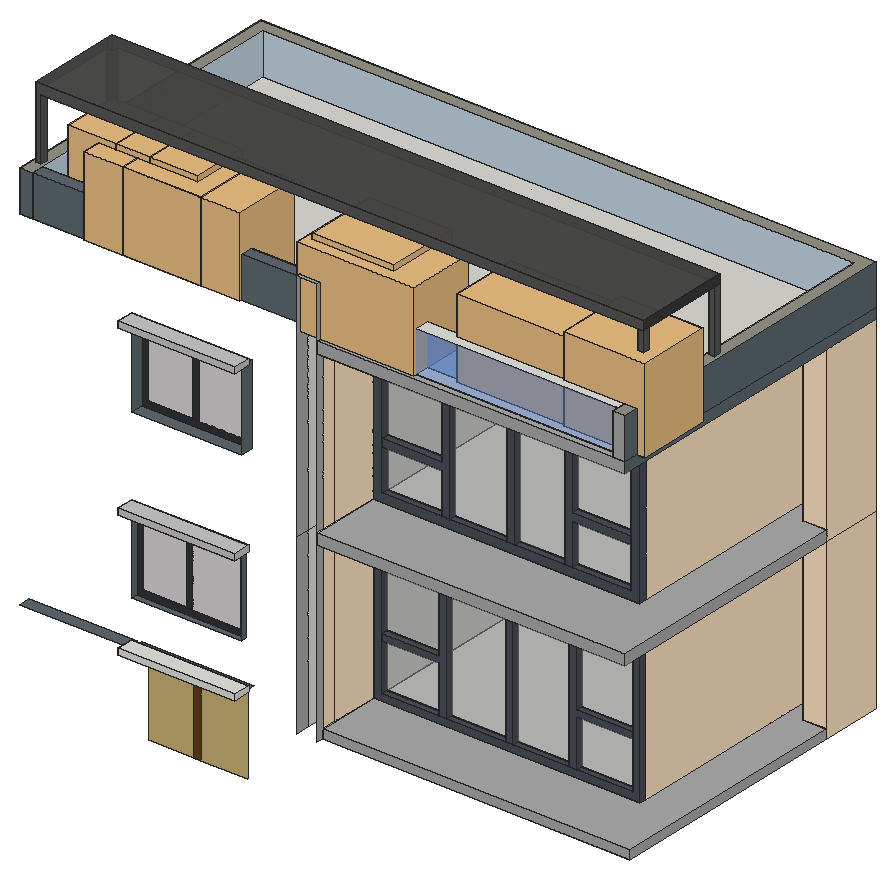
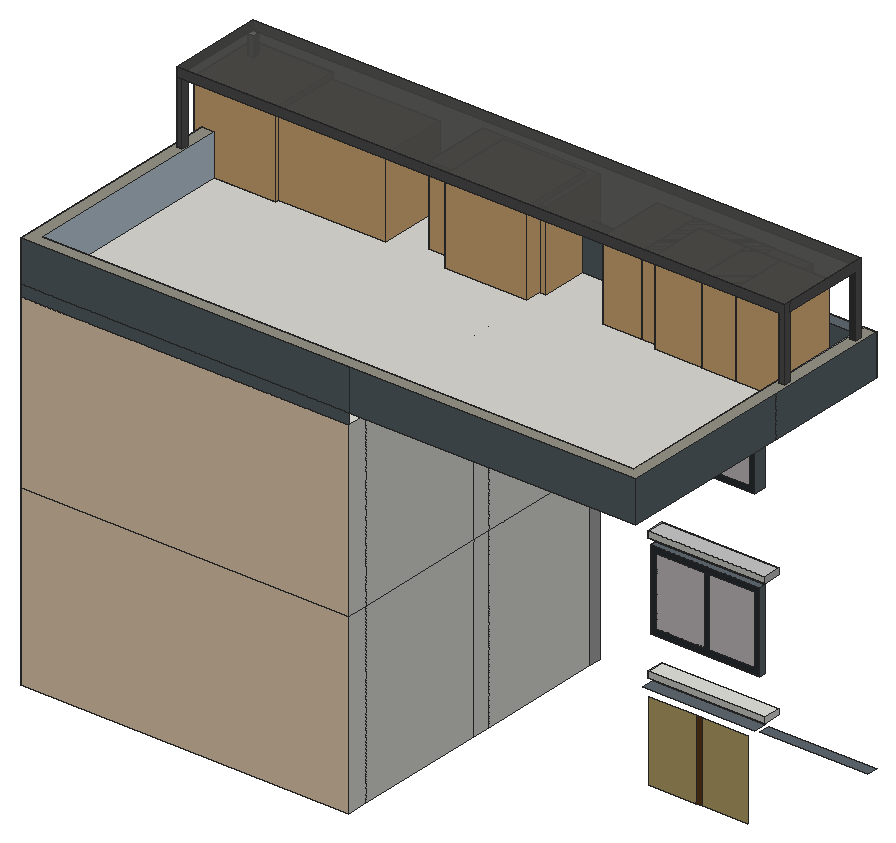
# SketchUp Ruby script. Lengths in inches.
U = 1.inch
M = Sketchup.active_model
def pt(a) = Geom::Point3d.new(a.map { |v| v * U })
def face(e, loops, mat)
  f = e.add_face(loops[0].map { |a| pt(a) })
  loops[1..].each { |l| e.add_face(l.map { |a| pt(a) }).erase! }
  f.material = f.back_material = mat if mat
  f
end
# faces: each face lists its corners as indices into pts; further lists are holes
def faces(e, pts, list, mat = nil) = list.each { |f| face(e, (f[0].is_a?(Array) ? f : [f]).map { |l| l.map { |i| pts[i] } }, mat) }
# xy, xz, yz: faces in a plane at the given z, y or x. An outline is a flat list of corners, or four numbers for a rectangle; further outlines are holes
def ring(l) = l.size == 4 ? [[l[0], l[1]], [l[2], l[1]], [l[2], l[3]], [l[0], l[3]]] : l.each_slice(2).to_a
def flat(e, list, mat, &to3) = list.each { |f| face(e, (f[0].is_a?(Array) ? f : [f]).map { |l| ring(l).map { |u, v| to3.(u, v) } }, mat) }
def xy(e, z, list, mat = nil) = flat(e, list, mat) { |x, y| [x, y, z] }
def xz(e, y, list, mat = nil) = flat(e, list, mat) { |x, z| [x, y, z] }
def yz(e, x, list, mat = nil) = flat(e, list, mat) { |y, z| [x, y, z] }
def lines(e, pts, list) = list.each { |a, b| e.add_line(pt(pts[a]), pt(pts[b])) }
# prism: a flat outline (further loops are holes) pulled along v
def prism(e, loops, v, mat = nil)
  f = face(e, loops, mat); d = Geom::Vector3d.new(v.map { |x| x * U })
  f.pushpull(f.normal.samedirection?(d) ? d.length : -d.length)
end
def box(e, o, s, mat = nil) = prism(e, [[o, [o[0] + s[0], o[1], o[2]], [o[0] + s[0], o[1] + s[1], o[2]], [o[0], o[1] + s[1], o[2]]]], [0, 0, s[2]], mat)
def at(x, y, z, deg = 0) = Geom::Transformation.translation(pt([x, y, z])) * Geom::Transformation.rotation(ORIGIN, Z_AXIS, deg.degrees)
def axes(o, x, y, z) = Geom::Transformation.new([*x, 0, *y, 0, *z, 0, *pt(o).to_a, 1])
def part(name) = M.definitions.add(name)
# library, detail: a bought-in or finely detailed component or shape, given as its bounding box
def library(name, o, s) = part(name).tap { |d| box(d.entities, o, s) }
def detail(e, o, s) = box(e.add_group.entities, o, s)
def put(e, d, t, mat = nil) = e.add_instance(d, t).tap { |i| i.material = mat if mat }
def group(e, t, mat = nil) = e.add_group.tap { |g| g.transformation = t; g.material = mat if mat }.entities
root = M.entities
M.materials.add("[0012_Bisque]").color = [255, 228, 196]
M.materials.add("[0035_Tan]").color = [210, 180, 140]
M.materials.add("[Blinds Cellular White]").color = [217, 211, 213]
M.materials.add("[Color M02]").color = [198, 198, 198]
M.materials.add("[Color M03]").color = [170, 170, 170]
M.materials.add("[Color M06]").color = [86, 86, 86]
M.materials.add("[Color M07]").color = [58, 58, 58]
M.materials.add("[Formica Graystone]1").color = [149, 146, 135]
M.materials.add("[Formica Laminate Dark]").color = [74, 78, 89]
M.materials.add("[Formica Speckled Grey]").color = [47, 53, 56]
M.materials.add("[Formica Speckled Grey]1").color = [94, 105, 111]
M.materials.add("[Terrazzo Light Blue]").color = [196, 214, 227]
M.materials.add("[Terrazzo Tile Light]").color = [219, 217, 210]
M.materials.add("[Translucent Glass Block Dark]1").color = [71, 71, 69]
M.materials["[Translucent Glass Block Dark]1"].alpha = 0.8
M.materials.add("[Translucent Glass Blue]").color = [100, 149, 237]
M.materials["[Translucent Glass Blue]"].alpha = 0.5
M.materials.add("[Translucent Glass Gray]1").color = [173, 173, 173]
M.materials["[Translucent Glass Gray]1"].alpha = 0.5
M.materials.add("[Window Covering 02]").color = [199, 178, 115]
M.materials.add("[Wood Floor Light]").color = [204, 176, 127]
M.materials.add("[Wood Floor Parquet]").color = [102, 62, 27]
M.materials.add("[Wood Floor]").color = [127, 86, 50]
c1 = library("chau cay",[-24.34,-109.24,0],[56.46,62.58,79.69])
c2 = library("Sem+nome",[-20.92,-6.25,0],[92.79,42.83,52.11])
box(root,[934.42,1163.08,1113.51],[394.37,58.44,20.12])
xy(root,972.31,[[2038.61,1644.77,2328.14,1674.71]],"[Wood Floor]")
xy(root,1077.79,[[1597.41,1197.49,1985.07,1247.68],[1597.41,1644.77,2438.87,2162.77]])
xy(root,1077.79,[[1985.07,1197.49,1985.07,1247.68,1597.41,1247.68,1597.41,1644.77,2438.87,1644.77,2438.87,2162.77,2570.48,2162.77,2570.48,2027.6,2634.5,2027.6,2634.5,1197.49]],"[0035_Tan]")
xy(root,1104.69,[[1597.41,1434.77,2496.41,2162.77],[2553.96,2027.6,2570.48,2162.77]])
xy(root,1106.33,[[1597.41,1413.09,2496.41,1434.77]])
xy(root,1106.33,[[1597.41,1197.49,2634.5,1197.49,2634.5,2027.6,2553.96,2027.6,2553.96,2162.77,2496.41,2162.77,2496.41,1413.09,1597.41,1413.09]],"[Color M03]")
xy(root,1108.67,[[560.3125,1221.52,922.73,1257.65],[937.5625,1221.52,1314.8125,1263.33]],"[Formica Speckled Grey]1")
xy(root,1129.41,[[1818.32,1413.09,1843.06,1434.77],[2042.55,1413.09,2067.28,1434.77],[2256.82,1413.09,2281.55,1434.77]])
xy(root,1129.41,[[1624.23,1413.09,1818.32,1434.77],[1843.06,1413.09,2042.55,1434.77],[2067.28,1413.09,2256.82,1434.77],[2281.55,1413.09,2469.59,1434.77]],"[Formica Laminate Dark]")
xy(root,1262.3,[[937.5625,1221.52,1307.26,1238.71]],"[Formica Speckled Grey]1")
xy(root,1288.71,[[1624.23,1413.09,1818.32,1434.77],[2281.55,1413.09,2469.59,1434.77]],"[Formica Laminate Dark]")
xy(root,1310.79,[[1624.23,1413.09,1818.32,1434.77],[2281.55,1413.09,2469.59,1434.77]],"[Formica Laminate Dark]")
xy(root,1522.7,[[1624.23,1413.09,1818.32,1434.77],[1843.06,1413.09,2042.55,1434.77],[2067.28,1413.09,2256.82,1434.77],[2281.55,1413.09,2469.59,1434.77]],"[Formica Laminate Dark]")
xy(root,1530.73,[[937.5625,1221.52,1307.26,1238.71]],"[Formica Speckled Grey]1")
xy(root,1536.95,[[934.42,1163.08,1328.79,1221.52]],"[Color M02]")
xy(root,1547.94,[[1624.23,1413.09,1818.32,1434.77],[1843.06,1413.09,2042.55,1434.77],[2067.28,1413.09,2256.82,1434.77],[2281.55,1413.09,2469.59,1434.77]],"[Formica Laminate Dark]")
xy(root,1557.07,[[934.42,1163.08,1328.79,1221.52]],"[Color M02]")
xy(root,1646.85,[[1818.32,1413.09,1843.06,1434.77],[2042.55,1413.09,2067.28,1434.77],[2256.82,1413.09,2281.55,1434.77]])
xy(root,1646.85,[[1624.23,1413.09,1818.32,1434.77],[1843.06,1413.09,2042.55,1434.77],[2067.28,1413.09,2256.82,1434.77],[2281.55,1413.09,2469.59,1434.77]],"[Formica Laminate Dark]")
xy(root,1671.57,[[1597.41,1413.09,2496.41,1434.77],[1597.41,1434.77,2496.41,2162.77]])
xy(root,1671.57,[[1597.41,1175.74,1597.41,1413.09,2496.41,1413.09,2496.41,2162.77,2553.96,2162.77,2553.96,2027.6,2634.5,2027.6,2634.5,1175.74]],"[0035_Tan]")
xy(root,1708.37,[[1597.41,1411.27,2496.41,1434.77],[1597.41,1434.77,2496.41,2162.77]])
xy(root,1708.37,[[1597.41,1175.74,2634.5,1175.74,2634.5,2027.6,2553.96,2027.6,2553.96,2162.77,2496.41,2162.77,2496.41,1411.27,1597.41,1411.27]],"[Color M03]")
xy(root,1736.45,[[1829.47,1411.27,1855.4,1434.77],[2047.9,1411.27,2073.84,1434.77],[2243.95,1411.27,2269.89,1434.77]])
xy(root,1736.45,[[1627.89,1411.27,1829.47,1434.77],[1855.4,1411.27,2047.9,1434.77],[2073.84,1411.27,2243.95,1434.77],[2269.89,1411.27,2465.9375,1434.77]],"[Formica Laminate Dark]")
xy(root,1822.8,[[937.5625,1221.52,1307.26,1262.83]],"[Formica Speckled Grey]1")
xy(root,1875.68,[[1627.89,1411.27,1829.47,1434.77],[2269.89,1411.27,2465.9375,1434.77]],"[Formica Laminate Dark]")
xy(root,1902.64,[[1627.89,1411.27,1829.47,1434.77],[2269.89,1411.27,2465.9375,1434.77]],"[Formica Laminate Dark]")
xy(root,2091.23,[[937.5625,1221.52,1307.26,1262.83]],"[Formica Speckled Grey]1")
xy(root,2100.86,[[1627.89,1411.27,1829.47,1434.77],[1855.4,1411.27,2047.9,1434.77],[2073.84,1411.27,2243.95,1434.77],[2269.89,1411.27,2465.9375,1434.77]],"[Formica Laminate Dark]")
xy(root,2101.01,[[934.42,1163.08,1328.79,1221.52]],"[Color M02]")
xy(root,2121.13,[[934.42,1163.08,1328.79,1221.52]],"[Color M02]")
xy(root,2123.1,[[1627.89,1411.27,1829.47,1434.77],[1855.4,1411.27,2047.9,1434.77],[2073.84,1411.27,2243.95,1434.77],[2269.89,1411.27,2465.9375,1434.77]],"[Formica Laminate Dark]")
xy(root,2222.77,[[1829.47,1411.27,1855.4,1434.77],[2047.9,1411.27,2073.84,1434.77],[2243.95,1411.27,2269.89,1434.77]])
xy(root,2222.77,[[1627.89,1411.27,1829.47,1434.77],[1855.4,1411.27,2047.9,1434.77],[2073.84,1411.27,2243.95,1434.77],[2269.89,1411.27,2465.9375,1434.77]],"[Formica Laminate Dark]")
xy(root,2250.85,[[1529,1256.68,1597.41,1434.77],[1597.41,1411.27,2496.41,1434.77],[1529,1434.77,1597.41,2234.7],[1597.41,1434.77,2496.41,2162.77],[2553.96,2027.6,2634.5,2234.7],
  [1597.41,2162.77,2438.87,2234.7],[2438.87,2162.77,2496.41,2234.7],[2496.41,2162.77,2553.96,2234.7]])
xy(root,2250.85,[[1597.41,1175.74,1597.41,1411.27,2496.41,1411.27,2496.41,2162.77,2553.96,2162.77,2553.96,2027.6,2634.5,2027.6,2634.5,1175.74]],"[0035_Tan]")
xy(root,2288.72,[[2592.99,1175.74,2592.99,2193.19,601.82,2193.19,601.82,1221.52,560.3125,1221.52,560.3125,2234.7,2634.5,2234.7,2634.5,1175.74],[1597.41,1197.49,2592.99,1243.8125],[601.82,1221.52,1529,1263.03],[1529,1247.68,1597.41,1256.68]])
xy(root,2288.72,[[1597.41,1175.74,2592.99,1197.49]],"[Color M03]")
xy(root,2288.72,[[1597.41,1243.8125,2592.99,1243.8125,2592.99,2193.19,601.82,2193.19,601.82,1263.03,1529,1263.03,1529,1256.68,1597.41,1256.68]],"[Terrazzo Tile Light]")
xy(root,2427.41,[[1597.41,1197.49,2592.99,1243.8125],[571.02,1271.52,590.77,1294.27],[2601.14,1271.52,2620.89,1294.27],[571.02,1571.45,590.77,1594.2],[2601.14,1571.45,2620.89,1594.2]])
xy(root,2427.41,[[[2592.99,1175.74,2634.5,1175.74,2634.5,2234.7,560.3125,2234.7,560.3125,1221.52,601.82,1221.52,601.82,2193.19,2592.99,2193.19],[2601.14,1271.52,2620.89,1294.27],[2601.14,1571.45,2620.89,1594.2],[571.02,1571.45,590.77,1594.2],[571.02,1271.52,590.77,1294.27]]],"[Formica Graystone]1")
xy(root,2427.41,[[601.82,1221.52,1529,1263.03]],"[Formica Speckled Grey]1")
xy(root,2461.1,[[1529,1175.74,1597.41,1247.68]],"[Color M03]")
xy(root,2636.87,[[2601.14,1271.52,2620.89,1294.27],[2601.14,1571.45,2620.89,1594.2]])
xy(root,2636.87,[[590.77,1271.52,590.77,1294.27,571.02,1294.27,571.02,1571.45,590.77,1571.45,590.77,1594.2,2601.14,1594.2,2601.14,1571.45,2620.89,1571.45,2620.89,1294.27,2601.14,1294.27,2601.14,1271.52]],"[Translucent Glass Block Dark]1")
xy(root,2667.72,[[571.02,1271.52,2620.89,1594.2]],"[Translucent Glass Block Dark]1")
xz(root,1163.08,[[934.42,1536.95,1328.79,1557.07],[934.42,2101.01,1328.79,2121.13]],"[Color M02]")
xz(root,1175.74,[[1597.41,1671.57,2634.5,1708.37],[1597.41,2250.85,2634.5,2288.72],[2592.99,2288.72,2634.5,2427.41]],"[Color M03]")
xz(root,1197.49,[[2586.03,2288.72,2592.99,2427.41]])
xz(root,1197.49,[[1597.41,1077.79,2634.5,1106.33]],"[Color M03]")
xz(root,1197.49,[[1597.41,2288.72,2586.03,2427.41]],"[Translucent Glass Blue]")
xz(root,1221.52,[[934.42,1536.95,1328.79,1557.07],[934.42,2101.01,1328.79,2121.13]])
xz(root,1221.52,[[560.3125,2288.72,601.82,2427.41],[601.82,2288.72,1529,2427.41]],"[Formica Speckled Grey]1")
xz(root,1238.71,[[958.89,1283.625,1106.3,1509.4],[1127,1283.625,1285.9375,1509.4]],"[Blinds Cellular White]")
xz(root,1238.71,[[[937.5625,1262.3,1307.26,1530.73],[958.89,1283.625,1285.9375,1509.4]],[1106.3,1283.625,1127,1509.4]],"[Formica Speckled Grey]")
xz(root,1243.8125,[[1597.41,2288.72,2592.99,2427.41]],"[Translucent Glass Blue]")
xz(root,1247.68,[[1529,2288.72,1597.41,2461.1]],"[Color M03]")
xz(root,1256.68,[[1529,2250.85,1597.41,2288.72]])
xz(root,1262.83,[[958.26,1843.5,1109,2070.53],[1133.75,1843.5,1286.57,2070.53]],"[Blinds Cellular White]")
xz(root,1262.83,[[[937.5625,1822.8,1307.26,2091.23],[958.26,1843.5,1286.57,2070.53]],[1109,1843.5,1133.75,2070.53]],"[Formica Speckled Grey]")
xz(root,1263.03,[[601.82,2288.72,1529,2427.41]],"[Formica Speckled Grey]1")
xz(root,1263.33,[[959.46,820.51,1112.13,1086.78],[1133.85,820.51,1292.91,1086.78]],"[Window Covering 02]")
xz(root,1263.33,[[1112.13,820.51,1133.85,1086.78]],"[Wood Floor Parquet]")
xz(root,1271.52,[[571.02,2427.41,590.77,2427.41,590.77,2636.87,2620.89,2636.87,2620.89,2667.72,571.02,2667.72],[2601.14,2427.41,2620.89,2636.87]],"[Color M06]")
xz(root,1294.27,[[2601.14,2427.41,2620.89,2636.87]])
xz(root,1294.27,[[571.02,2427.41,590.77,2636.87]],"[Color M07]")
xz(root,1411.27,[[[1597.41,1708.37,2496.41,2250.85],[1627.89,1736.45,2465.9375,2222.77]],[1829.47,1736.45,1855.4,1736.45,1855.4,2100.86,2047.9,2100.86,2047.9,1736.45,2073.84,1736.45,2073.84,2100.86,2243.95,2100.86,2243.95,1736.45,2269.89,1736.45,2269.89,1875.68,2465.9375,1875.68,2465.9375,1902.64,2269.89,1902.64,2269.89,2100.86,2465.9375,2100.86,2465.9375,2123.1,2269.89,2123.1,2269.89,2222.77,2243.95,2222.77,2243.95,2123.1,2073.84,2123.1,2073.84,2222.77,2047.9,2222.77,2047.9,2123.1,1855.4,2123.1,1855.4,2222.77,1829.47,2222.77,1829.47,2123.1,1627.89,2123.1,1627.89,2100.86,1829.47,2100.86,1829.47,1902.64,1627.89,1902.64,1627.89,1875.68,1829.47,1875.68]],"[Formica Laminate Dark]")
xz(root,1413.09,[[[1597.41,1106.33,2496.41,1671.57],[1624.23,1129.41,2469.59,1646.85]],[1818.32,1129.41,1843.06,1129.41,1843.06,1522.7,2042.55,1522.7,2042.55,1129.41,2067.28,1129.41,2067.28,1522.7,2256.82,1522.7,2256.82,1129.41,2281.55,1129.41,2281.55,1288.71,2469.59,1288.71,2469.59,1310.79,2281.55,1310.79,2281.55,1522.7,2469.59,1522.7,2469.59,1547.94,2281.55,1547.94,2281.55,1646.85,2256.82,1646.85,2256.82,1547.94,2067.28,1547.94,2067.28,1646.85,2042.55,1646.85,2042.55,1547.94,1843.06,1547.94,1843.06,1646.85,1818.32,1646.85,1818.32,1547.94,1624.23,1547.94,1624.23,1522.7,1818.32,1522.7,1818.32,1310.79,1624.23,1310.79,1624.23,1288.71,1818.32,1288.71]],"[Formica Laminate Dark]")
xz(root,1434.77,[[1597.41,1104.69,2496.41,1106.33],[[1597.41,1106.33,2496.41,1671.57],[1624.23,1129.41,2469.59,1646.85]],[1818.32,1129.41,1818.32,1288.71,1624.23,1288.71,1624.23,1310.79,1818.32,1310.79,1818.32,1522.7,1624.23,1522.7,1624.23,1547.94,1818.32,1547.94,1818.32,1646.85,1843.06,1646.85,1843.06,1547.94,2042.55,1547.94,2042.55,1646.85,2067.28,1646.85,2067.28,1547.94,2256.82,1547.94,2256.82,1646.85,2281.55,1646.85,2281.55,1547.94,2469.59,1547.94,2469.59,1522.7,2281.55,1522.7,2281.55,1310.79,2469.59,1310.79,2469.59,1288.71,2281.55,1288.71,2281.55,1129.41,2256.82,1129.41,2256.82,1522.7,2067.28,1522.7,2067.28,1129.41,2042.55,1129.41,2042.55,1522.7,1843.06,1522.7,1843.06,1129.41],[[1597.41,1708.37,2496.41,2250.85],[1627.89,1736.45,2465.9375,2222.77]],[1829.47,1736.45,1829.47,1875.68,1627.89,1875.68,1627.89,1902.64,1829.47,1902.64,1829.47,2100.86,1627.89,2100.86,1627.89,2123.1,1829.47,2123.1,1829.47,2222.77,1855.4,2222.77,1855.4,2123.1,2047.9,2123.1,2047.9,2222.77,2073.84,2222.77,2073.84,2123.1,2243.95,2123.1,2243.95,2222.77,2269.89,2222.77,2269.89,2123.1,2465.9375,2123.1,2465.9375,2100.86,2269.89,2100.86,2269.89,1902.64,2465.9375,1902.64,2465.9375,1875.68,2269.89,1875.68,2269.89,1736.45,2243.95,1736.45,2243.95,2100.86,2073.84,2100.86,2073.84,1736.45,2047.9,1736.45,2047.9,2100.86,1855.4,2100.86,1855.4,1736.45]])
xz(root,1434.77,[[1624.23,1129.41,1818.32,1288.71],[1843.06,1129.41,2042.55,1522.7],[2067.28,1129.41,2256.82,1522.7],[2281.55,1129.41,2469.59,1288.71],[1624.23,1310.79,1818.32,1522.7],
  [2281.55,1310.79,2469.59,1522.7],[1624.23,1547.94,1818.32,1646.85],[1843.06,1547.94,2042.55,1646.85],[2067.28,1547.94,2256.82,1646.85],[2281.55,1547.94,2469.59,1646.85],
  [1627.89,1736.45,1829.47,1875.68],[1855.4,1736.45,2047.9,2100.86],[2073.84,1736.45,2243.95,2100.86],[2269.89,1736.45,2465.9375,1875.68],[1627.89,1902.64,1829.47,2100.86],
  [2269.89,1902.64,2465.9375,2100.86],[1627.89,2123.1,1829.47,2222.77],[1855.4,2123.1,2047.9,2222.77],[2073.84,2123.1,2243.95,2222.77],[2269.89,2123.1,2465.9375,2222.77]],"[Translucent Glass Gray]1")
xz(root,1571.45,[[571.02,2427.41,590.77,2636.87],[2601.14,2427.41,2620.89,2636.87]],"[Color M06]")
xz(root,1594.2,[[571.02,2427.41,571.02,2667.72,2620.89,2667.72,2620.89,2636.87,590.77,2636.87,590.77,2427.41],[2601.14,2427.41,2620.89,2636.87]],"[Color M06]")
xz(root,2027.6,[[2570.48,1077.79,2634.5,1106.33],[2553.96,1104.69,2570.48,1106.33],[2553.96,1671.57,2634.5,1708.37]])
xz(root,2027.6,[[2553.96,1106.33,2634.5,1671.57],[2553.96,1708.37,2634.5,2250.85]],"[0012_Bisque]")
xz(root,2162.77,[[1597.41,1077.79,2438.87,1104.69],[2438.87,1077.79,2438.87,1104.69,2496.41,1104.69,2496.41,1106.33,2553.96,1106.33,2553.96,1104.69,2570.48,1104.69,2570.48,1077.79],[1597.41,1104.69,2438.87,1671.57],[2438.87,1104.69,2496.41,1671.57],[1597.41,1671.57,2438.87,1708.37],
  [2438.87,1671.57,2496.41,1708.37],[2496.41,1671.57,2553.96,1708.37],[1597.41,1708.37,2438.87,2250.85],[2438.87,1708.37,2496.41,2250.85]])
xz(root,2162.77,[[2496.41,1106.33,2553.96,1671.57],[2496.41,1708.37,2553.96,2250.85]],"[0012_Bisque]")
xz(root,2193.19,[[601.82,2288.72,2592.99,2427.41]],"[Terrazzo Light Blue]")
xz(root,2234.7,[[1529,1077.79,2634.5,1671.57],[1529,1671.57,2634.5,2250.85]],"[0012_Bisque]")
xz(root,2234.7,[[1529,2250.85,2634.5,2288.72],[560.3125,2288.72,1529,2427.41],[1529,2288.72,2634.5,2427.41]],"[Formica Speckled Grey]1")
yz(root,560.3125,[[1221.52,2288.72,1644.77,2427.41],[1644.77,2288.72,2234.7,2427.41]],"[Formica Speckled Grey]1")
yz(root,571.02,[[1271.52,2427.41,1271.52,2667.72,1571.45,2667.72,1571.45,2636.87,1294.27,2636.87,1294.27,2427.41],[1571.45,2427.41,1594.2,2667.72]],"[Color M06]")
yz(root,590.77,[[1271.52,2427.41,1294.27,2636.87],[1571.45,2427.41,1594.2,2636.87]],"[Color M06]")
yz(root,601.82,[[1221.52,2288.72,1263.03,2427.41]])
yz(root,601.82,[[1263.03,2288.72,1644.77,2427.41],[1644.77,2288.72,2193.19,2427.41]],"[Terrazzo Light Blue]")
yz(root,934.42,[[1163.08,1536.95,1221.52,1557.07],[1163.08,2101.01,1221.52,2121.13]],"[Color M02]")
yz(root,937.5625,[[1221.52,1262.3,1238.71,1530.73],[1221.52,1822.8,1262.83,2091.23]],"[Formica Speckled Grey]1")
yz(root,1307.26,[[1221.52,1262.3,1238.71,1530.73],[1221.52,1822.8,1262.83,2091.23]],"[Formica Speckled Grey]1")
yz(root,1328.79,[[1163.08,1536.95,1221.52,1557.07],[1163.08,2101.01,1221.52,2121.13]],"[Color M02]")
yz(root,1529,[[1221.52,1077.79,1644.77,1671.57],[1644.77,1077.79,1705.22,1671.57],[1705.22,1077.79,2162.77,1671.57],[2162.77,1077.79,2234.7,1671.57],[1221.52,1671.57,1644.77,1671.57,1644.77,2250.85,1256.68,2250.85,1256.68,2288.72,1221.52,2288.72],
  [1644.77,1671.57,1705.22,2250.85],[1705.22,1671.57,2162.77,2250.85],[2162.77,1671.57,2234.7,2250.85],[1221.52,2288.72,1247.68,2427.41],[1247.68,2288.72,1256.68,2427.41],
  [1256.68,2288.72,1263.03,2427.41]])
yz(root,1529,[[1175.74,1077.79,1221.52,1671.57],[1175.74,1671.57,1175.74,2461.1,1247.68,2461.1,1247.68,2427.41,1221.52,2427.41,1221.52,1671.57]],"[Color M03]")
yz(root,1597.41,[[1197.49,1077.79,1247.68,1106.33],[1247.68,1077.79,1247.68,1106.33,1434.77,1106.33,1434.77,1104.69,1644.77,1104.69,1644.77,1077.79],[1644.77,1077.79,2162.77,1104.69],[1434.77,1104.69,2162.77,1671.57],[1413.09,1106.33,1434.77,1671.57],
  [1175.74,1671.57,1247.68,1708.37],[1247.68,1671.57,1434.77,1708.37],[1434.77,1671.57,2162.77,1708.37],[1411.27,1708.37,1434.77,2250.85],[1434.77,1708.37,2162.77,2250.85],
  [1175.74,2250.85,1197.49,2288.72],[1197.49,2250.85,1247.68,2288.72],[1247.68,2250.85,1256.68,2288.72],[1197.49,2288.72,1243.8125,2427.41]])
yz(root,1597.41,[[1197.49,1106.33,1247.68,1671.57],[1247.68,1106.33,1413.09,1671.57],[1197.49,1708.37,1247.68,2250.85],[1247.68,1708.37,1411.27,2250.85]],"[0012_Bisque]")
yz(root,1597.41,[[1175.74,1077.79,1197.49,1671.57],[1175.74,1708.37,1197.49,2250.85],[1175.74,2288.72,1197.49,2461.1],[1243.8125,2288.72,1247.68,2288.72,1247.68,2461.1,1197.49,2461.1,1197.49,2427.41,1243.8125,2427.41]],"[Color M03]")
yz(root,1624.23,[[1413.09,1288.71,1434.77,1310.79],[1413.09,1522.7,1434.77,1547.94]])
yz(root,1624.23,[[1413.09,1129.41,1434.77,1288.71],[1413.09,1310.79,1434.77,1522.7],[1413.09,1547.94,1434.77,1646.85]],"[Formica Laminate Dark]")
yz(root,1627.89,[[1411.27,1875.68,1434.77,1902.64],[1411.27,2100.86,1434.77,2123.1]])
yz(root,1627.89,[[1411.27,1736.45,1434.77,1875.68],[1411.27,1902.64,1434.77,2100.86],[1411.27,2123.1,1434.77,2222.77]],"[Formica Laminate Dark]")
yz(root,1818.32,[[1413.09,1129.41,1434.77,1288.71],[1413.09,1310.79,1434.77,1522.7],[1413.09,1547.94,1434.77,1646.85]],"[Formica Laminate Dark]")
yz(root,1829.47,[[1411.27,1736.45,1434.77,1875.68],[1411.27,1902.64,1434.77,2100.86],[1411.27,2123.1,1434.77,2222.77]],"[Formica Laminate Dark]")
yz(root,1843.06,[[1413.09,1129.41,1434.77,1522.7],[1413.09,1547.94,1434.77,1646.85]],"[Formica Laminate Dark]")
yz(root,1855.4,[[1411.27,1736.45,1434.77,2100.86],[1411.27,2123.1,1434.77,2222.77]],"[Formica Laminate Dark]")
yz(root,2042.55,[[1413.09,1129.41,1434.77,1522.7],[1413.09,1547.94,1434.77,1646.85]],"[Formica Laminate Dark]")
yz(root,2047.9,[[1411.27,1736.45,1434.77,2100.86],[1411.27,2123.1,1434.77,2222.77]],"[Formica Laminate Dark]")
yz(root,2067.28,[[1413.09,1129.41,1434.77,1522.7],[1413.09,1547.94,1434.77,1646.85]],"[Formica Laminate Dark]")
yz(root,2073.84,[[1411.27,1736.45,1434.77,2100.86],[1411.27,2123.1,1434.77,2222.77]],"[Formica Laminate Dark]")
yz(root,2243.95,[[1411.27,1736.45,1434.77,2100.86],[1411.27,2123.1,1434.77,2222.77]],"[Formica Laminate Dark]")
yz(root,2256.82,[[1413.09,1129.41,1434.77,1522.7],[1413.09,1547.94,1434.77,1646.85]],"[Formica Laminate Dark]")
yz(root,2269.89,[[1411.27,1736.45,1434.77,1875.68],[1411.27,1902.64,1434.77,2100.86],[1411.27,2123.1,1434.77,2222.77]],"[Formica Laminate Dark]")
yz(root,2281.55,[[1413.09,1129.41,1434.77,1288.71],[1413.09,1310.79,1434.77,1522.7],[1413.09,1547.94,1434.77,1646.85]],"[Formica Laminate Dark]")
yz(root,2465.9375,[[1411.27,1875.68,1434.77,1902.64],[1411.27,2100.86,1434.77,2123.1]])
yz(root,2465.9375,[[1411.27,1736.45,1434.77,1875.68],[1411.27,1902.64,1434.77,2100.86],[1411.27,2123.1,1434.77,2222.77]],"[Formica Laminate Dark]")
yz(root,2469.59,[[1413.09,1288.71,1434.77,1310.79],[1413.09,1522.7,1434.77,1547.94]])
yz(root,2469.59,[[1413.09,1129.41,1434.77,1288.71],[1413.09,1310.79,1434.77,1522.7],[1413.09,1547.94,1434.77,1646.85]],"[Formica Laminate Dark]")
yz(root,2496.41,[[1434.77,1104.69,2162.77,1106.33]])
yz(root,2496.41,[[1434.77,1106.33,2162.77,1671.57],[1434.77,1708.37,2162.77,2250.85]],"[0012_Bisque]")
yz(root,2496.41,[[1413.09,1106.33,1434.77,1671.57],[1411.27,1708.37,1434.77,2250.85]],"[Formica Laminate Dark]")
yz(root,2553.96,[[2027.6,1104.69,2162.77,1106.33],[2027.6,1671.57,2162.77,1708.37]])
yz(root,2553.96,[[2027.6,1106.33,2162.77,1671.57],[2027.6,1708.37,2162.77,2250.85]],"[0012_Bisque]")
yz(root,2570.48,[[2027.6,1077.79,2162.77,1104.69]])
yz(root,2592.99,[[1197.49,2288.72,1243.8125,2427.41]])
yz(root,2592.99,[[1175.74,2288.72,1197.49,2427.41]],"[Color M03]")
yz(root,2592.99,[[1243.8125,2288.72,2193.19,2427.41]],"[Terrazzo Light Blue]")
yz(root,2601.14,[[1271.52,2427.41,1294.27,2636.87],[1571.45,2427.41,1594.2,2636.87]],"[Color M06]")
yz(root,2620.89,[[1271.52,2427.41,1294.27,2636.87],[1571.45,2427.41,1594.2,2636.87]],"[Color M06]")
yz(root,2620.89,[[1271.52,2636.87,1594.2,2667.72]],"[Color M07]")
yz(root,2634.5,[[2027.6,1077.79,2234.7,1671.57],[2027.6,1671.57,2234.7,2250.85]],"[0012_Bisque]")
yz(root,2634.5,[[1197.49,1077.79,2027.6,1106.33],[1175.74,1671.57,2027.6,1708.37]],"[Color M03]")
yz(root,2634.5,[[1175.74,2250.85,2234.7,2288.72],[1175.74,2288.72,2234.7,2427.41]],"[Formica Speckled Grey]1")
p = [[2078,1674.71,838.18],[2077.73,1674.71,836.07],[2077.73,1663.21,836.07],[2078,1663.21,838.18],[2094.04,1674.71,836.07],[2093.76,1674.71,838.18],
  [2093.76,1663.21,838.18],[2094.04,1663.21,836.07],[2078.82,1674.71,840.15],[2078.82,1663.21,840.15],[2092.95,1674.71,840.15],[2092.95,1663.21,840.15],
  [2080.12,1674.71,841.84],[2080.12,1663.21,841.84],[2091.65,1674.71,841.84],[2091.65,1663.21,841.84],[2081.8,1674.71,843.14],[2081.8,1663.21,843.14],
  [2089.96,1674.71,843.14],[2089.96,1663.21,843.14],[2083.77,1674.71,843.95],[2083.77,1663.21,843.95],[2087.99,1674.71,843.95],[2087.99,1663.21,843.95],
  [2085.88,1674.71,844.23],[2085.88,1663.21,844.23],[1529,1644.77,2250.85],[1529,1644.77,2288.72],[1529,1705.22,2250.85],[1529,1705.22,2288.72],
  [1529,2162.77,2250.85],[1529,2162.77,2288.72],[586.52,1571.45,2618.68],[586.52,1594.2,2618.68],[586.52,1571.45,2636.87],[586.52,1571.45,2642.6]]
faces(root,p,[[0,1,2,3],[4,5,6,7],[8,0,3,9],[5,10,11,6],[12,8,9,13],[10,14,15,11],[16,12,13,17],[14,18,19,15],
  [20,16,17,21],[18,22,23,19],[24,20,21,25],[22,24,25,23]],"[Wood Floor Light]")
lines(root,p,[[26,27],[28,29],[30,31],[32,33],[34,35]])
put(root,c1,axes([794.43,1606.42,2288.72],[4.876,0,0],[0,3,0],[0,0,3.55019]))
put(root,c1,axes([955.74,1606.42,2288.72],[4.876,0,0],[0,3,0],[0,0,3.55019]))
put(root,c2,axes([999.33,1249.79,2288.72],[4.23577,0,0],[0,5.31,0],[0,0,5.1072]))
put(root,c2,axes([867.46,1249.79,2288.72],[4.23577,0,0],[0,5.31,0],[0,0,5.1072]))
put(root,c2,axes([1607.21,1221.42,2288.72],[4.23577,0,0],[0,5.31,0],[0,0,5.1072]))
put(root,c2,axes([2110.89,1264.73,2288.72],[4.23577,0,0],[0,5.31,0],[0,0,5.1072]))
put(root,c1,axes([1658.11,1652.02,2288.72],[4.876,0,0],[0,3.9,0],[0,0,3.55019]))
put(root,c1,axes([2505.42,1652.02,2288.72],[4.876,0,0],[0,3.9,0],[0,0,3.55019]))
